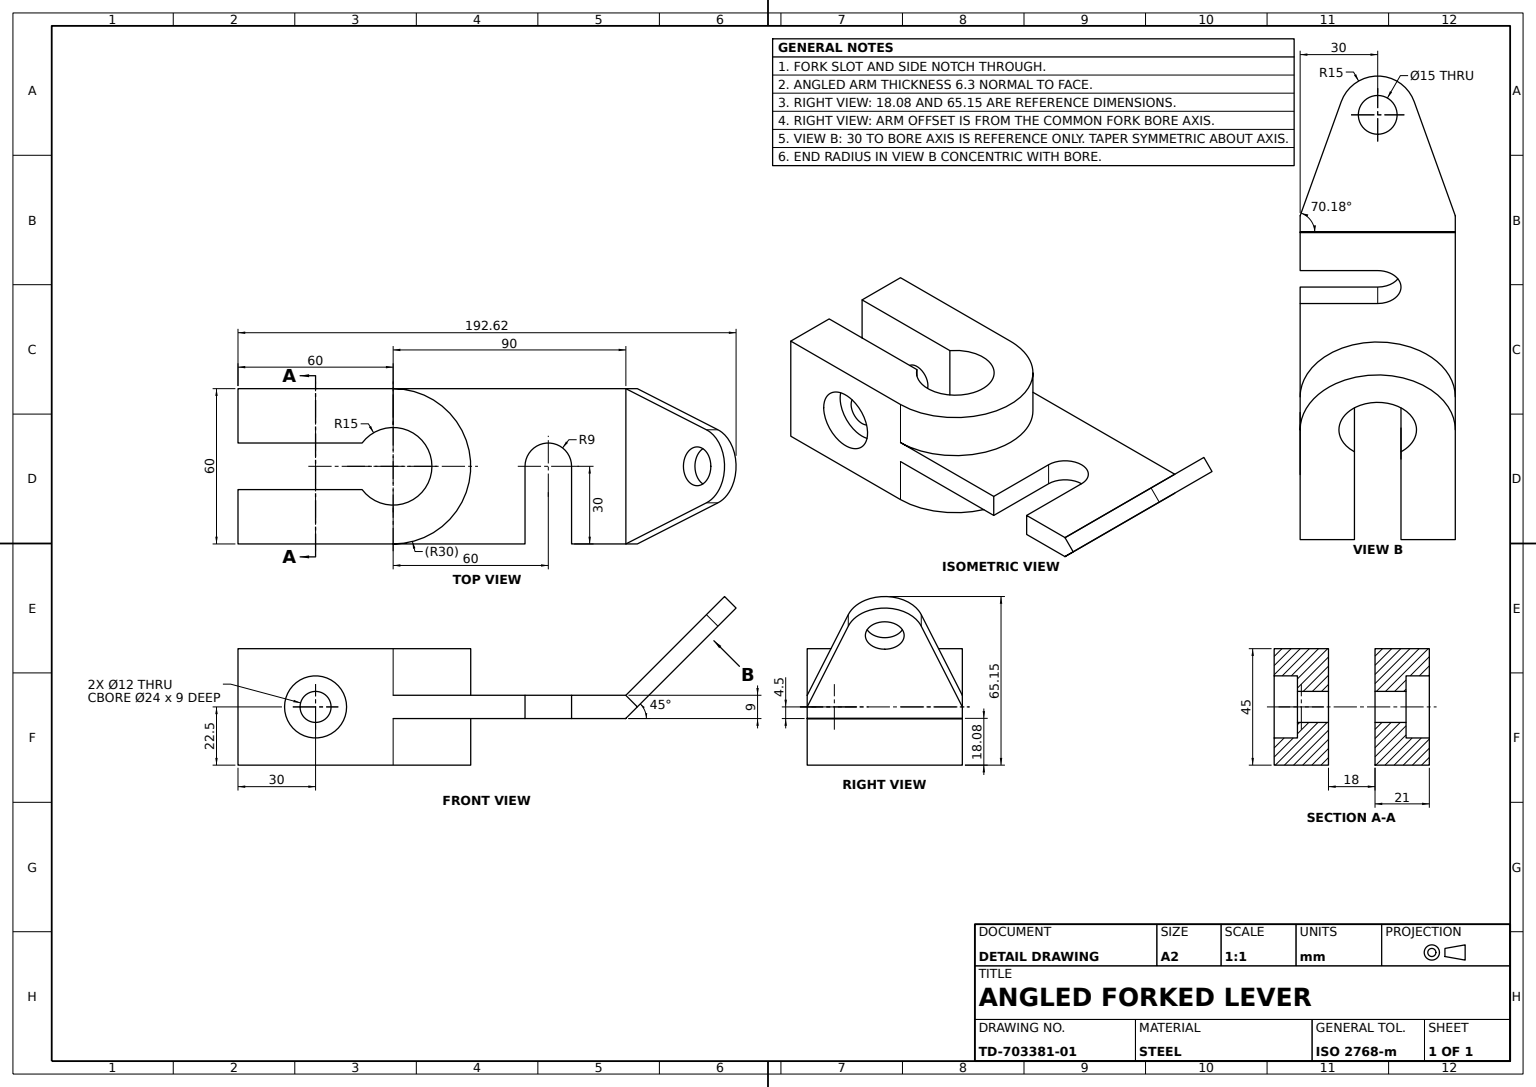
ISO-10303-21;
HEADER;
FILE_DESCRIPTION((''),'2;1');
FILE_NAME('','',(''),(''),'','','');
FILE_SCHEMA(('AUTOMOTIVE_DESIGN'));
ENDSEC;
DATA;
#1=APPLICATION_CONTEXT('');
#2=PRODUCT_CONTEXT('',#1,'mechanical');
#3=PRODUCT('','','',(#2));
#4=PRODUCT_DEFINITION_FORMATION('','',#3);
#5=PRODUCT_DEFINITION_CONTEXT('',#1,'design');
#6=PRODUCT_DEFINITION('','',#4,#5);
#7=PRODUCT_DEFINITION_SHAPE('','',#6);
#8=(LENGTH_UNIT()NAMED_UNIT(*)SI_UNIT(.MILLI.,.METRE.));
#9=(NAMED_UNIT(*)PLANE_ANGLE_UNIT()SI_UNIT($,.RADIAN.));
#10=(NAMED_UNIT(*)SI_UNIT($,.STERADIAN.)SOLID_ANGLE_UNIT());
#11=UNCERTAINTY_MEASURE_WITH_UNIT(LENGTH_MEASURE(0.005),#8,'distance_accuracy_value','');
#12=(GEOMETRIC_REPRESENTATION_CONTEXT(3)GLOBAL_UNCERTAINTY_ASSIGNED_CONTEXT((#11))GLOBAL_UNIT_ASSIGNED_CONTEXT((#8,#9,#10))REPRESENTATION_CONTEXT('',''));
#13=CARTESIAN_POINT('',(-30.,-30.,-22.5));
#14=VERTEX_POINT('',#13);
#15=CARTESIAN_POINT('',(-9.,-30.,-22.5));
#16=VERTEX_POINT('',#15);
#17=DIRECTION('',(1.,0.,0.));
#18=VECTOR('',#17,1000.);
#19=LINE('',#13,#18);
#20=EDGE_CURVE('',#14,#16,#19,.T.);
#21=ORIENTED_EDGE('',*,*,#20,.F.);
#22=CARTESIAN_POINT('',(-30.,30.,-22.5));
#23=VERTEX_POINT('',#22);
#24=DIRECTION('',(0.,-1.,0.));
#25=VECTOR('',#24,1000.);
#26=LINE('',#22,#25);
#27=EDGE_CURVE('',#23,#14,#26,.T.);
#28=ORIENTED_EDGE('',*,*,#27,.F.);
#29=CARTESIAN_POINT('',(30.,30.,-22.5));
#30=VERTEX_POINT('',#29);
#31=CARTESIAN_POINT('',(0.,30.,-22.5));
#32=DIRECTION('',(0.,0.,1.));
#33=AXIS2_PLACEMENT_3D('',#31,#32,#17);
#34=CIRCLE('',#33,30.);
#35=EDGE_CURVE('',#30,#23,#34,.T.);
#36=ORIENTED_EDGE('',*,*,#35,.F.);
#37=CARTESIAN_POINT('',(30.,-30.,-22.5));
#38=VERTEX_POINT('',#37);
#39=DIRECTION('',(0.,1.,0.));
#40=VECTOR('',#39,1000.);
#41=LINE('',#37,#40);
#42=EDGE_CURVE('',#38,#30,#41,.T.);
#43=ORIENTED_EDGE('',*,*,#42,.F.);
#44=CARTESIAN_POINT('',(9.,-30.,-22.5));
#45=VERTEX_POINT('',#44);
#46=EDGE_CURVE('',#45,#38,#19,.T.);
#47=ORIENTED_EDGE('',*,*,#46,.F.);
#48=CARTESIAN_POINT('',(9.,18.,-22.5));
#49=VERTEX_POINT('',#48);
#50=CARTESIAN_POINT('',(9.,30.,-22.5));
#51=LINE('',#50,#25);
#52=EDGE_CURVE('',#49,#45,#51,.T.);
#53=ORIENTED_EDGE('',*,*,#52,.F.);
#54=CARTESIAN_POINT('',(-9.,18.,-22.5));
#55=VERTEX_POINT('',#54);
#56=CIRCLE('',#33,15.);
#57=EDGE_CURVE('',#49,#55,#56,.T.);
#58=ORIENTED_EDGE('',*,*,#57,.T.);
#59=CARTESIAN_POINT('',(-9.,30.,-22.5));
#60=LINE('',#59,#40);
#61=EDGE_CURVE('',#16,#55,#60,.T.);
#62=ORIENTED_EDGE('',*,*,#61,.F.);
#63=EDGE_LOOP('',(#21,#28,#36,#43,#47,#53,#58,#62));
#64=FACE_BOUND('',#63,.T.);
#65=PLANE('',#33);
#66=ADVANCED_FACE('',(#64),#65,.F.);
#67=CARTESIAN_POINT('',(30.,30.,22.5));
#68=VERTEX_POINT('',#67);
#69=CARTESIAN_POINT('',(-30.,30.,22.5));
#70=VERTEX_POINT('',#69);
#71=CARTESIAN_POINT('',(0.,30.,22.5));
#72=AXIS2_PLACEMENT_3D('',#71,#32,#17);
#73=CIRCLE('',#72,30.);
#74=EDGE_CURVE('',#68,#70,#73,.T.);
#75=ORIENTED_EDGE('',*,*,#74,.F.);
#76=CARTESIAN_POINT('',(30.,30.,4.5));
#77=VERTEX_POINT('',#76);
#78=DIRECTION('',(0.,0.,-1.));
#79=VECTOR('',#78,1000.);
#80=LINE('',#67,#79);
#81=EDGE_CURVE('',#68,#77,#80,.T.);
#82=ORIENTED_EDGE('',*,*,#81,.T.);
#83=CARTESIAN_POINT('',(-30.,30.,4.5));
#84=VERTEX_POINT('',#83);
#85=CARTESIAN_POINT('',(0.,30.,4.5));
#86=DIRECTION('',(-1.,0.,0.));
#87=AXIS2_PLACEMENT_3D('',#85,#78,#86);
#88=CIRCLE('',#87,30.);
#89=EDGE_CURVE('',#84,#77,#88,.T.);
#90=ORIENTED_EDGE('',*,*,#89,.F.);
#91=LINE('',#69,#79);
#92=EDGE_CURVE('',#70,#84,#91,.T.);
#93=ORIENTED_EDGE('',*,*,#92,.F.);
#94=EDGE_LOOP('',(#75,#82,#90,#93));
#95=FACE_BOUND('',#94,.T.);
#96=AXIS2_PLACEMENT_3D('',#71,#78,#86);
#97=CYLINDRICAL_SURFACE('',#96,30.);
#98=ADVANCED_FACE('',(#95),#97,.T.);
#99=CARTESIAN_POINT('',(9.,-30.,22.5));
#100=VERTEX_POINT('',#99);
#101=VECTOR('',#32,1000.);
#102=LINE('',#99,#101);
#103=EDGE_CURVE('',#45,#100,#102,.T.);
#104=ORIENTED_EDGE('',*,*,#103,.T.);
#105=CARTESIAN_POINT('',(9.,18.,22.5));
#106=VERTEX_POINT('',#105);
#107=CARTESIAN_POINT('',(9.,30.,22.5));
#108=LINE('',#107,#25);
#109=EDGE_CURVE('',#106,#100,#108,.T.);
#110=ORIENTED_EDGE('',*,*,#109,.F.);
#111=LINE('',#105,#79);
#112=EDGE_CURVE('',#106,#49,#111,.T.);
#113=ORIENTED_EDGE('',*,*,#112,.T.);
#114=ORIENTED_EDGE('',*,*,#52,.T.);
#115=EDGE_LOOP('',(#104,#110,#113,#114));
#116=FACE_BOUND('',#115,.T.);
#117=CARTESIAN_POINT('',(9.,-6.,0.));
#118=VERTEX_POINT('',#117);
#119=CARTESIAN_POINT('',(9.,0.,0.));
#120=AXIS2_PLACEMENT_3D('',#119,#86,#24);
#121=CIRCLE('',#120,6.);
#122=EDGE_CURVE('',#118,#118,#121,.T.);
#123=ORIENTED_EDGE('',*,*,#122,.F.);
#124=EDGE_LOOP('',(#123));
#125=FACE_BOUND('',#124,.T.);
#126=CARTESIAN_POINT('',(9.,-34.105263,52.));
#127=AXIS2_PLACEMENT_3D('',#126,#86,#24);
#128=PLANE('',#127);
#129=ADVANCED_FACE('',(#116,#125),#128,.T.);
#130=CARTESIAN_POINT('',(-30.,119.838261,-4.579856));
#131=VERTEX_POINT('',#130);
#132=CARTESIAN_POINT('',(30.,119.838261,-4.579856));
#133=VERTEX_POINT('',#132);
#134=LINE('',#130,#18);
#135=EDGE_CURVE('',#131,#133,#134,.T.);
#136=ORIENTED_EDGE('',*,*,#135,.F.);
#137=CARTESIAN_POINT('',(-30.,119.918117,-4.5));
#138=VERTEX_POINT('',#137);
#139=CARTESIAN_POINT('',(-30.,124.434455,0.016338));
#140=DIRECTION('',(0.,-0.707106781,-0.707106781));
#141=VECTOR('',#140,1000.);
#142=LINE('',#139,#141);
#143=EDGE_CURVE('',#138,#131,#142,.T.);
#144=ORIENTED_EDGE('',*,*,#143,.F.);
#145=CARTESIAN_POINT('',(30.,119.918117,-4.5));
#146=VERTEX_POINT('',#145);
#147=CARTESIAN_POINT('',(0.,119.918117,-4.5));
#148=VECTOR('',#86,1000.);
#149=LINE('',#147,#148);
#150=EDGE_CURVE('',#146,#138,#149,.T.);
#151=ORIENTED_EDGE('',*,*,#150,.F.);
#152=DIRECTION('',(0.,0.707106781,0.707106781));
#153=VECTOR('',#152,1000.);
#154=LINE('',#132,#153);
#155=EDGE_CURVE('',#133,#146,#154,.T.);
#156=ORIENTED_EDGE('',*,*,#155,.F.);
#157=EDGE_LOOP('',(#136,#144,#151,#156));
#158=FACE_BOUND('',#157,.T.);
#159=CARTESIAN_POINT('',(0.,152.01162,27.593503));
#160=DIRECTION('',(0.,-0.707106781,0.707106781));
#161=AXIS2_PLACEMENT_3D('',#159,#160,#140);
#162=PLANE('',#161);
#163=ADVANCED_FACE('',(#158),#162,.F.);
#164=CARTESIAN_POINT('',(-30.,120.,-4.418117));
#165=VERTEX_POINT('',#164);
#166=CARTESIAN_POINT('',(30.,120.,-4.418117));
#167=VERTEX_POINT('',#166);
#168=LINE('',#164,#18);
#169=EDGE_CURVE('',#165,#167,#168,.T.);
#170=ORIENTED_EDGE('',*,*,#169,.F.);
#171=VERTEX_POINT('',#139);
#172=EDGE_CURVE('',#171,#165,#142,.T.);
#173=ORIENTED_EDGE('',*,*,#172,.F.);
#174=CARTESIAN_POINT('',(-14.111514,155.607809,31.189693));
#175=VERTEX_POINT('',#174);
#176=DIRECTION('',(-0.339052021,-0.665223168,-0.665223168));
#177=VECTOR('',#176,1000.);
#178=LINE('',#174,#177);
#179=EDGE_CURVE('',#175,#171,#178,.T.);
#180=ORIENTED_EDGE('',*,*,#179,.F.);
#181=CARTESIAN_POINT('',(14.111514,155.607809,31.189693));
#182=VERTEX_POINT('',#181);
#183=AXIS2_PLACEMENT_3D('',#159,#160,#17);
#184=CIRCLE('',#183,15.);
#185=EDGE_CURVE('',#182,#175,#184,.T.);
#186=ORIENTED_EDGE('',*,*,#185,.F.);
#187=CARTESIAN_POINT('',(30.,124.434455,0.016338));
#188=VERTEX_POINT('',#187);
#189=DIRECTION('',(-0.339052021,0.665223168,0.665223168));
#190=VECTOR('',#189,1000.);
#191=LINE('',#187,#190);
#192=EDGE_CURVE('',#188,#182,#191,.T.);
#193=ORIENTED_EDGE('',*,*,#192,.F.);
#194=EDGE_CURVE('',#167,#188,#154,.T.);
#195=ORIENTED_EDGE('',*,*,#194,.F.);
#196=EDGE_LOOP('',(#170,#173,#180,#186,#193,#195));
#197=FACE_BOUND('',#196,.T.);
#198=CARTESIAN_POINT('',(0.,146.708319,22.290202));
#199=VERTEX_POINT('',#198);
#200=CIRCLE('',#161,7.5);
#201=EDGE_CURVE('',#199,#199,#200,.T.);
#202=ORIENTED_EDGE('',*,*,#201,.T.);
#203=EDGE_LOOP('',(#202));
#204=FACE_BOUND('',#203,.T.);
#205=ADVANCED_FACE('',(#197,#204),#162,.F.);
#206=CARTESIAN_POINT('',(30.,-12.,0.));
#207=VERTEX_POINT('',#206);
#208=CARTESIAN_POINT('',(30.,0.,0.));
#209=AXIS2_PLACEMENT_3D('',#208,#86,#24);
#210=CIRCLE('',#209,12.);
#211=EDGE_CURVE('',#207,#207,#210,.T.);
#212=ORIENTED_EDGE('',*,*,#211,.T.);
#213=EDGE_LOOP('',(#212));
#214=FACE_BOUND('',#213,.T.);
#215=CARTESIAN_POINT('',(30.,81.,-4.5));
#216=VERTEX_POINT('',#215);
#217=CARTESIAN_POINT('',(30.,81.,4.5));
#218=VERTEX_POINT('',#217);
#219=CARTESIAN_POINT('',(30.,81.,22.5));
#220=LINE('',#219,#101);
#221=EDGE_CURVE('',#216,#218,#220,.T.);
#222=ORIENTED_EDGE('',*,*,#221,.T.);
#223=CARTESIAN_POINT('',(30.,120.,4.5));
#224=LINE('',#223,#25);
#225=EDGE_CURVE('',#218,#77,#224,.T.);
#226=ORIENTED_EDGE('',*,*,#225,.T.);
#227=ORIENTED_EDGE('',*,*,#81,.F.);
#228=CARTESIAN_POINT('',(30.,-30.,22.5));
#229=VERTEX_POINT('',#228);
#230=LINE('',#228,#40);
#231=EDGE_CURVE('',#229,#68,#230,.T.);
#232=ORIENTED_EDGE('',*,*,#231,.F.);
#233=LINE('',#228,#79);
#234=EDGE_CURVE('',#229,#38,#233,.T.);
#235=ORIENTED_EDGE('',*,*,#234,.T.);
#236=ORIENTED_EDGE('',*,*,#42,.T.);
#237=CARTESIAN_POINT('',(30.,30.,-4.5));
#238=VERTEX_POINT('',#237);
#239=EDGE_CURVE('',#238,#30,#80,.T.);
#240=ORIENTED_EDGE('',*,*,#239,.F.);
#241=CARTESIAN_POINT('',(30.,120.,-4.5));
#242=LINE('',#241,#25);
#243=EDGE_CURVE('',#216,#238,#242,.T.);
#244=ORIENTED_EDGE('',*,*,#243,.F.);
#245=EDGE_LOOP('',(#222,#226,#227,#232,#235,#236,#240,#244));
#246=FACE_BOUND('',#245,.T.);
#247=AXIS2_PLACEMENT_3D('',#228,#86,#24);
#248=PLANE('',#247);
#249=ADVANCED_FACE('',(#214,#246),#248,.F.);
#250=CARTESIAN_POINT('',(-30.,12.,0.));
#251=VERTEX_POINT('',#250);
#252=CARTESIAN_POINT('',(-30.,0.,0.));
#253=AXIS2_PLACEMENT_3D('',#252,#17,#39);
#254=CIRCLE('',#253,12.);
#255=EDGE_CURVE('',#251,#251,#254,.T.);
#256=ORIENTED_EDGE('',*,*,#255,.F.);
#257=EDGE_LOOP('',(#256));
#258=FACE_BOUND('',#257,.T.);
#259=CARTESIAN_POINT('',(-21.,12.,0.));
#260=VERTEX_POINT('',#259);
#261=CARTESIAN_POINT('',(-21.,0.,0.));
#262=AXIS2_PLACEMENT_3D('',#261,#17,#39);
#263=CIRCLE('',#262,12.);
#264=EDGE_CURVE('',#260,#260,#263,.T.);
#265=ORIENTED_EDGE('',*,*,#264,.T.);
#266=EDGE_LOOP('',(#265));
#267=FACE_BOUND('',#266,.T.);
#268=CYLINDRICAL_SURFACE('',#253,12.);
#269=ADVANCED_FACE('',(#258,#267),#268,.F.);
#270=CARTESIAN_POINT('',(-9.,6.,0.));
#271=VERTEX_POINT('',#270);
#272=CARTESIAN_POINT('',(-9.,0.,0.));
#273=AXIS2_PLACEMENT_3D('',#272,#17,#39);
#274=CIRCLE('',#273,6.);
#275=EDGE_CURVE('',#271,#271,#274,.T.);
#276=ORIENTED_EDGE('',*,*,#275,.F.);
#277=EDGE_LOOP('',(#276));
#278=FACE_BOUND('',#277,.T.);
#279=CARTESIAN_POINT('',(-9.,-30.,22.5));
#280=VERTEX_POINT('',#279);
#281=CARTESIAN_POINT('',(-9.,18.,22.5));
#282=VERTEX_POINT('',#281);
#283=CARTESIAN_POINT('',(-9.,30.,22.5));
#284=LINE('',#283,#40);
#285=EDGE_CURVE('',#280,#282,#284,.T.);
#286=ORIENTED_EDGE('',*,*,#285,.F.);
#287=LINE('',#279,#79);
#288=EDGE_CURVE('',#280,#16,#287,.T.);
#289=ORIENTED_EDGE('',*,*,#288,.T.);
#290=ORIENTED_EDGE('',*,*,#61,.T.);
#291=LINE('',#281,#79);
#292=EDGE_CURVE('',#55,#282,#291,.F.);
#293=ORIENTED_EDGE('',*,*,#292,.T.);
#294=EDGE_LOOP('',(#286,#289,#290,#293));
#295=FACE_BOUND('',#294,.T.);
#296=CARTESIAN_POINT('',(-9.,29.368421,52.));
#297=AXIS2_PLACEMENT_3D('',#296,#17,#39);
#298=PLANE('',#297);
#299=ADVANCED_FACE('',(#278,#295),#298,.T.);
#300=CARTESIAN_POINT('',(0.,99.,-4.5));
#301=VERTEX_POINT('',#300);
#302=CARTESIAN_POINT('',(0.,99.,4.5));
#303=VERTEX_POINT('',#302);
#304=CARTESIAN_POINT('',(0.,99.,52.));
#305=LINE('',#304,#79);
#306=EDGE_CURVE('',#301,#303,#305,.F.);
#307=ORIENTED_EDGE('',*,*,#306,.F.);
#308=CARTESIAN_POINT('',(30.,99.,-4.5));
#309=VERTEX_POINT('',#308);
#310=LINE('',#300,#18);
#311=EDGE_CURVE('',#301,#309,#310,.T.);
#312=ORIENTED_EDGE('',*,*,#311,.T.);
#313=CARTESIAN_POINT('',(30.,99.,4.5));
#314=VERTEX_POINT('',#313);
#315=CARTESIAN_POINT('',(30.,99.,22.5));
#316=LINE('',#315,#79);
#317=EDGE_CURVE('',#314,#309,#316,.T.);
#318=ORIENTED_EDGE('',*,*,#317,.F.);
#319=LINE('',#302,#18);
#320=EDGE_CURVE('',#303,#314,#319,.T.);
#321=ORIENTED_EDGE('',*,*,#320,.F.);
#322=EDGE_LOOP('',(#307,#312,#318,#321));
#323=FACE_BOUND('',#322,.T.);
#324=AXIS2_PLACEMENT_3D('',#304,#39,#32);
#325=PLANE('',#324);
#326=ADVANCED_FACE('',(#323),#325,.F.);
#327=ORIENTED_EDGE('',*,*,#225,.F.);
#328=CARTESIAN_POINT('',(0.,81.,4.5));
#329=VERTEX_POINT('',#328);
#330=LINE('',#328,#148);
#331=EDGE_CURVE('',#218,#329,#330,.T.);
#332=ORIENTED_EDGE('',*,*,#331,.T.);
#333=CARTESIAN_POINT('',(0.,90.,4.5));
#334=AXIS2_PLACEMENT_3D('',#333,#78,#86);
#335=CIRCLE('',#334,9.);
#336=EDGE_CURVE('',#329,#303,#335,.T.);
#337=ORIENTED_EDGE('',*,*,#336,.T.);
#338=ORIENTED_EDGE('',*,*,#320,.T.);
#339=VERTEX_POINT('',#223);
#340=EDGE_CURVE('',#339,#314,#224,.T.);
#341=ORIENTED_EDGE('',*,*,#340,.F.);
#342=CARTESIAN_POINT('',(-30.,120.,4.5));
#343=VERTEX_POINT('',#342);
#344=LINE('',#342,#18);
#345=EDGE_CURVE('',#343,#339,#344,.T.);
#346=ORIENTED_EDGE('',*,*,#345,.F.);
#347=LINE('',#83,#40);
#348=EDGE_CURVE('',#84,#343,#347,.T.);
#349=ORIENTED_EDGE('',*,*,#348,.F.);
#350=ORIENTED_EDGE('',*,*,#89,.T.);
#351=EDGE_LOOP('',(#327,#332,#337,#338,#341,#346,#349,#350));
#352=FACE_BOUND('',#351,.T.);
#353=CARTESIAN_POINT('',(0.,0.,4.5));
#354=AXIS2_PLACEMENT_3D('',#353,#78,#86);
#355=PLANE('',#354);
#356=ADVANCED_FACE('',(#352),#355,.F.);
#357=CARTESIAN_POINT('',(-30.,120.,-4.5));
#358=VERTEX_POINT('',#357);
#359=VERTEX_POINT('',#241);
#360=LINE('',#357,#18);
#361=EDGE_CURVE('',#358,#359,#360,.T.);
#362=ORIENTED_EDGE('',*,*,#361,.F.);
#363=LINE('',#342,#79);
#364=EDGE_CURVE('',#165,#358,#363,.T.);
#365=ORIENTED_EDGE('',*,*,#364,.F.);
#366=ORIENTED_EDGE('',*,*,#169,.T.);
#367=LINE('',#223,#79);
#368=EDGE_CURVE('',#167,#359,#367,.T.);
#369=ORIENTED_EDGE('',*,*,#368,.T.);
#370=EDGE_LOOP('',(#362,#365,#366,#369));
#371=FACE_BOUND('',#370,.T.);
#372=AXIS2_PLACEMENT_3D('',#342,#39,#32);
#373=PLANE('',#372);
#374=ADVANCED_FACE('',(#371),#373,.T.);
#375=CARTESIAN_POINT('',(30.,119.758405,-4.5));
#376=VERTEX_POINT('',#375);
#377=CARTESIAN_POINT('',(-30.,119.758405,-4.5));
#378=VERTEX_POINT('',#377);
#379=CARTESIAN_POINT('',(0.,119.758405,-4.5));
#380=LINE('',#379,#148);
#381=EDGE_CURVE('',#376,#378,#380,.T.);
#382=ORIENTED_EDGE('',*,*,#381,.T.);
#383=VECTOR('',#160,1000.);
#384=LINE('',#130,#383);
#385=EDGE_CURVE('',#131,#378,#384,.T.);
#386=ORIENTED_EDGE('',*,*,#385,.F.);
#387=ORIENTED_EDGE('',*,*,#135,.T.);
#388=LINE('',#132,#383);
#389=EDGE_CURVE('',#133,#376,#388,.T.);
#390=ORIENTED_EDGE('',*,*,#389,.T.);
#391=EDGE_LOOP('',(#382,#386,#387,#390));
#392=FACE_BOUND('',#391,.T.);
#393=DIRECTION('',(0.,0.707106781,-0.707106781));
#394=AXIS2_PLACEMENT_3D('',#130,#140,#393);
#395=PLANE('',#394);
#396=ADVANCED_FACE('',(#392),#395,.T.);
#397=ORIENTED_EDGE('',*,*,#255,.T.);
#398=EDGE_LOOP('',(#397));
#399=FACE_BOUND('',#398,.T.);
#400=ORIENTED_EDGE('',*,*,#172,.T.);
#401=ORIENTED_EDGE('',*,*,#364,.T.);
#402=CARTESIAN_POINT('',(-30.,30.,-4.5));
#403=LINE('',#402,#40);
#404=EDGE_CURVE('',#138,#358,#403,.T.);
#405=ORIENTED_EDGE('',*,*,#404,.F.);
#406=ORIENTED_EDGE('',*,*,#143,.T.);
#407=ORIENTED_EDGE('',*,*,#385,.T.);
#408=VERTEX_POINT('',#402);
#409=EDGE_CURVE('',#408,#378,#403,.T.);
#410=ORIENTED_EDGE('',*,*,#409,.F.);
#411=EDGE_CURVE('',#408,#23,#91,.T.);
#412=ORIENTED_EDGE('',*,*,#411,.T.);
#413=ORIENTED_EDGE('',*,*,#27,.T.);
#414=CARTESIAN_POINT('',(-30.,-30.,22.5));
#415=VERTEX_POINT('',#414);
#416=LINE('',#414,#79);
#417=EDGE_CURVE('',#415,#14,#416,.T.);
#418=ORIENTED_EDGE('',*,*,#417,.F.);
#419=LINE('',#69,#25);
#420=EDGE_CURVE('',#70,#415,#419,.T.);
#421=ORIENTED_EDGE('',*,*,#420,.F.);
#422=ORIENTED_EDGE('',*,*,#92,.T.);
#423=ORIENTED_EDGE('',*,*,#348,.T.);
#424=CARTESIAN_POINT('',(-30.,120.,4.450793));
#425=VERTEX_POINT('',#424);
#426=EDGE_CURVE('',#343,#425,#363,.T.);
#427=ORIENTED_EDGE('',*,*,#426,.T.);
#428=LINE('',#139,#383);
#429=EDGE_CURVE('',#171,#425,#428,.T.);
#430=ORIENTED_EDGE('',*,*,#429,.F.);
#431=EDGE_LOOP('',(#400,#401,#405,#406,#407,#410,#412,#413,#418,#421,#422,#423,#427,#430));
#432=FACE_BOUND('',#431,.T.);
#433=AXIS2_PLACEMENT_3D('',#69,#17,#39);
#434=PLANE('',#433);
#435=ADVANCED_FACE('',(#399,#432),#434,.F.);
#436=LINE('',#414,#18);
#437=EDGE_CURVE('',#415,#280,#436,.T.);
#438=ORIENTED_EDGE('',*,*,#437,.F.);
#439=ORIENTED_EDGE('',*,*,#417,.T.);
#440=ORIENTED_EDGE('',*,*,#20,.T.);
#441=ORIENTED_EDGE('',*,*,#288,.F.);
#442=EDGE_LOOP('',(#438,#439,#440,#441));
#443=FACE_BOUND('',#442,.T.);
#444=AXIS2_PLACEMENT_3D('',#414,#39,#32);
#445=PLANE('',#444);
#446=ADVANCED_FACE('',(#443),#445,.F.);
#447=CARTESIAN_POINT('',(-14.111514,151.153037,35.644465));
#448=VERTEX_POINT('',#447);
#449=LINE('',#174,#383);
#450=EDGE_CURVE('',#175,#448,#449,.T.);
#451=ORIENTED_EDGE('',*,*,#450,.F.);
#452=ORIENTED_EDGE('',*,*,#179,.T.);
#453=ORIENTED_EDGE('',*,*,#429,.T.);
#454=CARTESIAN_POINT('',(-29.989644,120.,4.491429));
#455=VERTEX_POINT('',#454);
#456=CARTESIAN_POINT('',(-29.988225,120.,4.496999));
#457=DIRECTION('',(0.246948062,0.,0.969028717));
#458=VECTOR('',#457,1000.);
#459=LINE('',#456,#458);
#460=EDGE_CURVE('',#425,#455,#459,.T.);
#461=ORIENTED_EDGE('',*,*,#460,.T.);
#462=LINE('',#447,#177);
#463=EDGE_CURVE('',#448,#455,#462,.T.);
#464=ORIENTED_EDGE('',*,*,#463,.F.);
#465=EDGE_LOOP('',(#451,#452,#453,#461,#464));
#466=FACE_BOUND('',#465,.T.);
#467=DIRECTION('',(-0.940767627,0.239745983,0.239745983));
#468=AXIS2_PLACEMENT_3D('',#174,#467,#457);
#469=PLANE('',#468);
#470=ADVANCED_FACE('',(#466),#469,.T.);
#471=ORIENTED_EDGE('',*,*,#74,.T.);
#472=ORIENTED_EDGE('',*,*,#420,.T.);
#473=ORIENTED_EDGE('',*,*,#437,.T.);
#474=ORIENTED_EDGE('',*,*,#285,.T.);
#475=CIRCLE('',#96,15.);
#476=EDGE_CURVE('',#282,#106,#475,.T.);
#477=ORIENTED_EDGE('',*,*,#476,.T.);
#478=ORIENTED_EDGE('',*,*,#109,.T.);
#479=EDGE_CURVE('',#100,#229,#436,.T.);
#480=ORIENTED_EDGE('',*,*,#479,.T.);
#481=ORIENTED_EDGE('',*,*,#231,.T.);
#482=EDGE_LOOP('',(#471,#472,#473,#474,#477,#478,#480,#481));
#483=FACE_BOUND('',#482,.T.);
#484=PLANE('',#72);
#485=ADVANCED_FACE('',(#483),#484,.T.);
#486=ORIENTED_EDGE('',*,*,#192,.T.);
#487=CARTESIAN_POINT('',(14.111514,151.153037,35.644465));
#488=VERTEX_POINT('',#487);
#489=LINE('',#181,#383);
#490=EDGE_CURVE('',#182,#488,#489,.T.);
#491=ORIENTED_EDGE('',*,*,#490,.T.);
#492=CARTESIAN_POINT('',(29.989644,120.,4.491429));
#493=VERTEX_POINT('',#492);
#494=CARTESIAN_POINT('',(30.,119.979682,4.471111));
#495=LINE('',#494,#190);
#496=EDGE_CURVE('',#493,#488,#495,.T.);
#497=ORIENTED_EDGE('',*,*,#496,.F.);
#498=CARTESIAN_POINT('',(30.,120.,4.450793));
#499=VERTEX_POINT('',#498);
#500=CARTESIAN_POINT('',(26.329224,120.,18.854985));
#501=DIRECTION('',(0.246948062,0.,-0.969028717));
#502=VECTOR('',#501,1000.);
#503=LINE('',#500,#502);
#504=EDGE_CURVE('',#493,#499,#503,.T.);
#505=ORIENTED_EDGE('',*,*,#504,.T.);
#506=LINE('',#187,#383);
#507=EDGE_CURVE('',#188,#499,#506,.T.);
#508=ORIENTED_EDGE('',*,*,#507,.F.);
#509=EDGE_LOOP('',(#486,#491,#497,#505,#508));
#510=FACE_BOUND('',#509,.T.);
#511=DIRECTION('',(0.940767627,0.239745983,0.239745983));
#512=AXIS2_PLACEMENT_3D('',#187,#511,#501);
#513=PLANE('',#512);
#514=ADVANCED_FACE('',(#510),#513,.T.);
#515=ORIENTED_EDGE('',*,*,#211,.F.);
#516=EDGE_LOOP('',(#515));
#517=FACE_BOUND('',#516,.T.);
#518=CARTESIAN_POINT('',(21.,-12.,0.));
#519=VERTEX_POINT('',#518);
#520=CARTESIAN_POINT('',(21.,0.,0.));
#521=AXIS2_PLACEMENT_3D('',#520,#86,#24);
#522=CIRCLE('',#521,12.);
#523=EDGE_CURVE('',#519,#519,#522,.F.);
#524=ORIENTED_EDGE('',*,*,#523,.F.);
#525=EDGE_LOOP('',(#524));
#526=FACE_BOUND('',#525,.T.);
#527=CYLINDRICAL_SURFACE('',#209,12.);
#528=ADVANCED_FACE('',(#517,#526),#527,.F.);
#529=ORIENTED_EDGE('',*,*,#57,.F.);
#530=ORIENTED_EDGE('',*,*,#112,.F.);
#531=ORIENTED_EDGE('',*,*,#476,.F.);
#532=ORIENTED_EDGE('',*,*,#292,.F.);
#533=EDGE_LOOP('',(#529,#530,#531,#532));
#534=FACE_BOUND('',#533,.T.);
#535=CYLINDRICAL_SURFACE('',#96,15.);
#536=ADVANCED_FACE('',(#534),#535,.F.);
#537=CARTESIAN_POINT('',(0.,152.860148,37.351576));
#538=VERTEX_POINT('',#537);
#539=CARTESIAN_POINT('',(0.,147.556847,32.048276));
#540=AXIS2_PLACEMENT_3D('',#539,#393,#152);
#541=CIRCLE('',#540,7.5);
#542=EDGE_CURVE('',#538,#538,#541,.T.);
#543=ORIENTED_EDGE('',*,*,#542,.F.);
#544=EDGE_LOOP('',(#543));
#545=FACE_BOUND('',#544,.T.);
#546=ORIENTED_EDGE('',*,*,#201,.F.);
#547=EDGE_LOOP('',(#546));
#548=FACE_BOUND('',#547,.T.);
#549=CYLINDRICAL_SURFACE('',#540,7.5);
#550=ADVANCED_FACE('',(#545,#548),#549,.F.);
#551=CARTESIAN_POINT('',(-30.,120.,4.491429));
#552=LINE('',#551,#18);
#553=EDGE_CURVE('',#455,#493,#552,.T.);
#554=ORIENTED_EDGE('',*,*,#553,.F.);
#555=ORIENTED_EDGE('',*,*,#460,.F.);
#556=ORIENTED_EDGE('',*,*,#426,.F.);
#557=ORIENTED_EDGE('',*,*,#345,.T.);
#558=EDGE_CURVE('',#339,#499,#367,.T.);
#559=ORIENTED_EDGE('',*,*,#558,.T.);
#560=ORIENTED_EDGE('',*,*,#504,.F.);
#561=EDGE_LOOP('',(#554,#555,#556,#557,#559,#560));
#562=FACE_BOUND('',#561,.T.);
#563=ADVANCED_FACE('',(#562),#373,.T.);
#564=ORIENTED_EDGE('',*,*,#311,.F.);
#565=CARTESIAN_POINT('',(0.,81.,-4.5));
#566=VERTEX_POINT('',#565);
#567=CARTESIAN_POINT('',(0.,90.,-4.5));
#568=AXIS2_PLACEMENT_3D('',#567,#78,#86);
#569=CIRCLE('',#568,9.);
#570=EDGE_CURVE('',#566,#301,#569,.T.);
#571=ORIENTED_EDGE('',*,*,#570,.F.);
#572=LINE('',#565,#148);
#573=EDGE_CURVE('',#216,#566,#572,.T.);
#574=ORIENTED_EDGE('',*,*,#573,.F.);
#575=ORIENTED_EDGE('',*,*,#243,.T.);
#576=CARTESIAN_POINT('',(0.,30.,-4.5));
#577=AXIS2_PLACEMENT_3D('',#576,#78,#86);
#578=CIRCLE('',#577,30.);
#579=EDGE_CURVE('',#408,#238,#578,.T.);
#580=ORIENTED_EDGE('',*,*,#579,.F.);
#581=ORIENTED_EDGE('',*,*,#409,.T.);
#582=ORIENTED_EDGE('',*,*,#381,.F.);
#583=EDGE_CURVE('',#376,#309,#242,.T.);
#584=ORIENTED_EDGE('',*,*,#583,.T.);
#585=EDGE_LOOP('',(#564,#571,#574,#575,#580,#581,#582,#584));
#586=FACE_BOUND('',#585,.T.);
#587=CARTESIAN_POINT('',(0.,0.,-4.5));
#588=AXIS2_PLACEMENT_3D('',#587,#78,#86);
#589=PLANE('',#588);
#590=ADVANCED_FACE('',(#586),#589,.T.);
#591=ORIENTED_EDGE('',*,*,#479,.F.);
#592=ORIENTED_EDGE('',*,*,#103,.F.);
#593=ORIENTED_EDGE('',*,*,#46,.T.);
#594=ORIENTED_EDGE('',*,*,#234,.F.);
#595=EDGE_LOOP('',(#591,#592,#593,#594));
#596=FACE_BOUND('',#595,.T.);
#597=ADVANCED_FACE('',(#596),#445,.F.);
#598=ORIENTED_EDGE('',*,*,#523,.T.);
#599=EDGE_LOOP('',(#598));
#600=FACE_BOUND('',#599,.T.);
#601=CARTESIAN_POINT('',(21.,-6.,0.));
#602=VERTEX_POINT('',#601);
#603=CIRCLE('',#521,6.);
#604=EDGE_CURVE('',#602,#602,#603,.F.);
#605=ORIENTED_EDGE('',*,*,#604,.F.);
#606=EDGE_LOOP('',(#605));
#607=FACE_BOUND('',#606,.T.);
#608=PLANE('',#521);
#609=ADVANCED_FACE('',(#600,#607),#608,.F.);
#610=ORIENTED_EDGE('',*,*,#450,.T.);
#611=AXIS2_PLACEMENT_3D('',#539,#160,#17);
#612=CIRCLE('',#611,15.);
#613=EDGE_CURVE('',#488,#448,#612,.T.);
#614=ORIENTED_EDGE('',*,*,#613,.F.);
#615=ORIENTED_EDGE('',*,*,#490,.F.);
#616=ORIENTED_EDGE('',*,*,#185,.T.);
#617=EDGE_LOOP('',(#610,#614,#615,#616));
#618=FACE_BOUND('',#617,.T.);
#619=CYLINDRICAL_SURFACE('',#161,15.);
#620=ADVANCED_FACE('',(#618),#619,.T.);
#621=CARTESIAN_POINT('',(-21.,6.,0.));
#622=VERTEX_POINT('',#621);
#623=CIRCLE('',#262,6.);
#624=EDGE_CURVE('',#622,#622,#623,.T.);
#625=ORIENTED_EDGE('',*,*,#624,.T.);
#626=EDGE_LOOP('',(#625));
#627=FACE_BOUND('',#626,.T.);
#628=ORIENTED_EDGE('',*,*,#264,.F.);
#629=EDGE_LOOP('',(#628));
#630=FACE_BOUND('',#629,.T.);
#631=PLANE('',#262);
#632=ADVANCED_FACE('',(#627,#630),#631,.F.);
#633=ORIENTED_EDGE('',*,*,#306,.T.);
#634=ORIENTED_EDGE('',*,*,#336,.F.);
#635=CARTESIAN_POINT('',(0.,81.,52.));
#636=LINE('',#635,#79);
#637=EDGE_CURVE('',#566,#329,#636,.F.);
#638=ORIENTED_EDGE('',*,*,#637,.F.);
#639=ORIENTED_EDGE('',*,*,#570,.T.);
#640=EDGE_LOOP('',(#633,#634,#638,#639));
#641=FACE_BOUND('',#640,.T.);
#642=CARTESIAN_POINT('',(0.,90.,52.));
#643=AXIS2_PLACEMENT_3D('',#642,#78,#86);
#644=CYLINDRICAL_SURFACE('',#643,9.);
#645=ADVANCED_FACE('',(#641),#644,.F.);
#646=ORIENTED_EDGE('',*,*,#411,.F.);
#647=ORIENTED_EDGE('',*,*,#579,.T.);
#648=ORIENTED_EDGE('',*,*,#239,.T.);
#649=ORIENTED_EDGE('',*,*,#35,.T.);
#650=EDGE_LOOP('',(#646,#647,#648,#649));
#651=FACE_BOUND('',#650,.T.);
#652=ADVANCED_FACE('',(#651),#97,.T.);
#653=ORIENTED_EDGE('',*,*,#361,.T.);
#654=EDGE_CURVE('',#359,#146,#242,.T.);
#655=ORIENTED_EDGE('',*,*,#654,.T.);
#656=ORIENTED_EDGE('',*,*,#150,.T.);
#657=ORIENTED_EDGE('',*,*,#404,.T.);
#658=EDGE_LOOP('',(#653,#655,#656,#657));
#659=FACE_BOUND('',#658,.T.);
#660=ADVANCED_FACE('',(#659),#589,.T.);
#661=ORIENTED_EDGE('',*,*,#542,.T.);
#662=EDGE_LOOP('',(#661));
#663=FACE_BOUND('',#662,.T.);
#664=ORIENTED_EDGE('',*,*,#463,.T.);
#665=ORIENTED_EDGE('',*,*,#553,.T.);
#666=ORIENTED_EDGE('',*,*,#496,.T.);
#667=ORIENTED_EDGE('',*,*,#613,.T.);
#668=EDGE_LOOP('',(#664,#665,#666,#667));
#669=FACE_BOUND('',#668,.T.);
#670=AXIS2_PLACEMENT_3D('',#539,#160,#140);
#671=PLANE('',#670);
#672=ADVANCED_FACE('',(#663,#669),#671,.T.);
#673=ORIENTED_EDGE('',*,*,#624,.F.);
#674=EDGE_LOOP('',(#673));
#675=FACE_BOUND('',#674,.T.);
#676=ORIENTED_EDGE('',*,*,#275,.T.);
#677=EDGE_LOOP('',(#676));
#678=FACE_BOUND('',#677,.T.);
#679=CARTESIAN_POINT('',(95.383414,0.,0.));
#680=AXIS2_PLACEMENT_3D('',#679,#17,#39);
#681=CYLINDRICAL_SURFACE('',#680,6.);
#682=ADVANCED_FACE('',(#675,#678),#681,.F.);
#683=ORIENTED_EDGE('',*,*,#583,.F.);
#684=ORIENTED_EDGE('',*,*,#389,.F.);
#685=ORIENTED_EDGE('',*,*,#155,.T.);
#686=ORIENTED_EDGE('',*,*,#654,.F.);
#687=ORIENTED_EDGE('',*,*,#368,.F.);
#688=ORIENTED_EDGE('',*,*,#194,.T.);
#689=ORIENTED_EDGE('',*,*,#507,.T.);
#690=ORIENTED_EDGE('',*,*,#558,.F.);
#691=ORIENTED_EDGE('',*,*,#340,.T.);
#692=ORIENTED_EDGE('',*,*,#317,.T.);
#693=EDGE_LOOP('',(#683,#684,#685,#686,#687,#688,#689,#690,#691,#692));
#694=FACE_BOUND('',#693,.T.);
#695=ADVANCED_FACE('',(#694),#248,.F.);
#696=ORIENTED_EDGE('',*,*,#573,.T.);
#697=ORIENTED_EDGE('',*,*,#637,.T.);
#698=ORIENTED_EDGE('',*,*,#331,.F.);
#699=ORIENTED_EDGE('',*,*,#221,.F.);
#700=EDGE_LOOP('',(#696,#697,#698,#699));
#701=FACE_BOUND('',#700,.T.);
#702=CARTESIAN_POINT('',(34.,81.,52.));
#703=AXIS2_PLACEMENT_3D('',#702,#24,#78);
#704=PLANE('',#703);
#705=ADVANCED_FACE('',(#701),#704,.F.);
#706=ORIENTED_EDGE('',*,*,#122,.T.);
#707=EDGE_LOOP('',(#706));
#708=FACE_BOUND('',#707,.T.);
#709=ORIENTED_EDGE('',*,*,#604,.T.);
#710=EDGE_LOOP('',(#709));
#711=FACE_BOUND('',#710,.T.);
#712=CARTESIAN_POINT('',(-95.383414,0.,0.));
#713=AXIS2_PLACEMENT_3D('',#712,#86,#24);
#714=CYLINDRICAL_SURFACE('',#713,6.);
#715=ADVANCED_FACE('',(#708,#711),#714,.F.);
#716=CLOSED_SHELL('',(#66,#98,#129,#163,#205,#249,#269,#299,#326,#356,#374,#396,#435,#446,#470,#485,#514,#528,#536,#550,#563,#590,#597,#609,#620,#632,#645,#652,#660,#672,#682,#695,#705,#715));
#717=MANIFOLD_SOLID_BREP('',#716);
#718=ADVANCED_BREP_SHAPE_REPRESENTATION('',(#717),#12);
#719=SHAPE_DEFINITION_REPRESENTATION(#7,#718);
ENDSEC;
END-ISO-10303-21;
